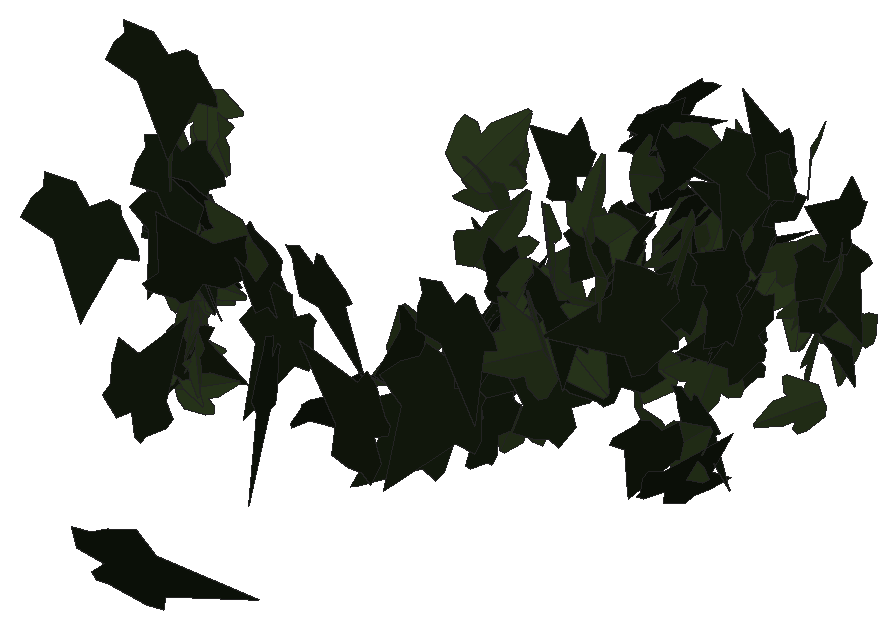
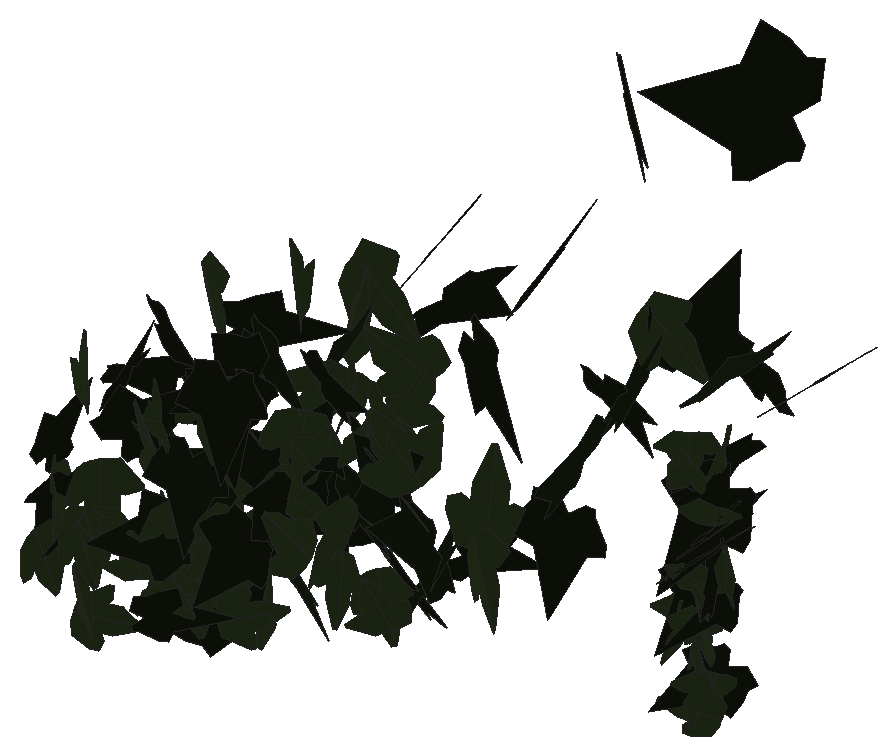
# SketchUp Ruby script. Lengths in inches.
U = 1.inch
M = Sketchup.active_model
def pt(a) = Geom::Point3d.new(a.map { |v| v * U })
def face(e, loops, mat)
  f = e.add_face(loops[0].map { |a| pt(a) })
  loops[1..].each { |l| e.add_face(l.map { |a| pt(a) }).erase! }
  f.material = f.back_material = mat if mat
  f
end
# faces: each face lists its corners as indices into pts; further lists are holes
def faces(e, pts, list, mat = nil) = list.each { |f| face(e, (f[0].is_a?(Array) ? f : [f]).map { |l| l.map { |i| pts[i] } }, mat) }
# xy, xz, yz: faces in a plane at the given z, y or x. An outline is a flat list of corners, or four numbers for a rectangle; further outlines are holes
def ring(l) = l.size == 4 ? [[l[0], l[1]], [l[2], l[1]], [l[2], l[3]], [l[0], l[3]]] : l.each_slice(2).to_a
def flat(e, list, mat, &to3) = list.each { |f| face(e, (f[0].is_a?(Array) ? f : [f]).map { |l| ring(l).map { |u, v| to3.(u, v) } }, mat) }
def xy(e, z, list, mat = nil) = flat(e, list, mat) { |x, y| [x, y, z] }
def xz(e, y, list, mat = nil) = flat(e, list, mat) { |x, z| [x, y, z] }
def yz(e, x, list, mat = nil) = flat(e, list, mat) { |y, z| [x, y, z] }
def lines(e, pts, list) = list.each { |a, b| e.add_line(pt(pts[a]), pt(pts[b])) }
# prism: a flat outline (further loops are holes) pulled along v
def prism(e, loops, v, mat = nil)
  f = face(e, loops, mat); d = Geom::Vector3d.new(v.map { |x| x * U })
  f.pushpull(f.normal.samedirection?(d) ? d.length : -d.length)
end
def box(e, o, s, mat = nil) = prism(e, [[o, [o[0] + s[0], o[1], o[2]], [o[0] + s[0], o[1] + s[1], o[2]], [o[0], o[1] + s[1], o[2]]]], [0, 0, s[2]], mat)
def at(x, y, z, deg = 0) = Geom::Transformation.translation(pt([x, y, z])) * Geom::Transformation.rotation(ORIGIN, Z_AXIS, deg.degrees)
def axes(o, x, y, z) = Geom::Transformation.new([*x, 0, *y, 0, *z, 0, *pt(o).to_a, 1])
def part(name) = M.definitions.add(name)
# library, detail: a bought-in or finely detailed component or shape, given as its bounding box
def library(name, o, s) = part(name).tap { |d| box(d.entities, o, s) }
def detail(e, o, s) = box(e.add_group.entities, o, s)
def put(e, d, t, mat = nil) = e.add_instance(d, t).tap { |i| i.material = mat if mat }
def group(e, t, mat = nil) = e.add_group.tap { |g| g.transformation = t; g.material = mat if mat }.entities
root = M.entities
M.materials.add("efeu1").color = [18, 25, 13]
M.materials.add("efeu2").color = [43, 57, 29]
c1 = part("ivyleaf_9")
p = [[1.54,2.16,1.25],[1.36,2.04,1.19],[-0.21,0.99,0.68],[-0.71,1.11,0.82],[-0.85,0.86,0.67],[-0.8,0.17,0.21],
  [-0.9,-0.01,0.1],[-0.67,-0.16,-0.02],[-0.08,-0.08,-0.05],[-0.03,-0.6,-0.4],[0.65,-0.88,-0.66],[0.83,-0.6,-0.49],
  [1.29,-0.42,-0.43],[1.8125,-0.07,-0.26],[1.21,0.44,0.15]]
faces(c1.entities,p,[[0,1,2,3,4,5,6,7,8,9,10,11,12,13,14]],"efeu1")
c2 = part("ivyleaf_10")
p = [[0,0.5,-0.03],[-0.0625,2.02,-0.43],[-0.19,2.01,-0.46],[-0.54,1.05,-0.29],[-0.52,0.625,-0.18],[-0.83,0.76,-0.28],
  [-1.16,0.64,-0.33],[-1.15,0.33,-0.24],[-0.77,-0.39,0.02],[-0.3,-0.51,0.16],[0.04,-0.48,0.23],[-0.02,2.01,-0.4375],
  [-0.06,2.01,-0.43],[0.04,-0.49,0.23],[0.67,-0.49,0.14],[1.38,0.36,-0.2],[1.375,0.51,-0.24],[0.81,0.65,-0.19],
  [0.62,0.59,-0.15],[0.6,1.09,-0.28],[0.5,1.23,-0.31]]
faces(c2.entities,p,[[0,1,2,3,4,5,6,7,8,9,10],[11,12,0,13,14,15,16,17,18,19,20]],"efeu2")
put(root,c1,axes([597.06,111.03,169.78],[0.8884,-0.27376,1.03511],[1.04614,-0.06449,-0.91492],[0.22801,1.36255,0.16467]))
put(root,c1,axes([597.32,117.23,172.98],[-0.66463,0.21669,-1.02259],[0.98764,-0.26673,-0.69844],[-0.34238,-1.19008,-0.02966]))
put(root,c1,axes([590.51,120.16,168.07],[-0.54205,0.57536,0.71293],[0.49254,-0.51545,0.79047],[0.77247,0.73239,-0.00375]))
put(root,c1,axes([597.17,121.51,169.04],[0.02116,-1.10176,0.25788],[0.00386,0.25799,1.10193],[-1.13153,-0.01973,0.00858]))
put(root,c1,axes([586.375,123.42,170.97],[-0.15788,-1.13606,0.27735],[0.27693,-0.30823,-1.10489],[1.13616,-0.08274,0.30785]))
put(root,c1,axes([590.33,123.15,170.4375],[0.56967,0.20223,0.80165],[-0.7533,-0.27424,0.60449],[0.34072,-0.94444,-0.00387]))
put(root,c1,axes([598,123.75,169.59],[-0.48576,-0.91416,0.37838],[-0.19107,-0.32691,-1.0351],[0.97074,-0.52179,-0.0144]))
put(root,c1,axes([597.72,124.3,171.68],[0.29974,-1.04193,0.1721],[0.06502,-0.16035,-1.08404],[1.05405,0.30619,0.01793]))
put(root,c2,axes([591.05,123.89,171.4375],[-0.49829,-0.14247,0.83957],[-0.81301,-0.20983,-0.51813],[0.25337,-0.95349,-0.01142]))
put(root,c1,axes([592.26,124.37,169.37],[-0.90433,-0.11689,-0.34199],[0.33902,0.04499,-0.91186],[0.12525,-0.96579,-0.00109]))
put(root,c1,axes([590.61,124.88,170.59],[0.86227,-0.73938,-0.36016],[-0.2705,0.23783,-1.13586],[0.77668,0.9037,0.00426]))
put(root,c1,axes([596.14,124.86,169.32],[0.048,0.03236,-1.17542],[-1.17289,-0.08233,-0.05016],[-0.08361,1.17352,0.02889]))
put(root,c2,axes([599.42,125.35,170.56],[-0.55467,-0.00306,0.99705],[-0.98974,-0.13623,-0.55103],[0.12053,-1.13279,0.06358]))
put(root,c1,axes([592.125,126.17,166.32],[0.24002,0.89785,0.01121],[0.00274,0.01087,-0.92938],[-0.89792,0.24003,0.00015]))
put(root,c2,axes([598.72,126.74,169.57],[-0.75092,0.65629,-0.00469],[-0.01407,-0.00897,0.99717],[0.65616,0.75088,0.01601]))
put(root,c1,axes([585.61,127.62,173.34],[-0.08041,-1.08649,0.38625],[0.35343,-0.39177,-1.02845],[1.0976,0.04655,0.35946]))
put(root,c1,axes([586,127.66,168.86],[-0.16927,-0.80439,0.33478],[-0.0648,-0.32847,-0.82199],[0.86886,-0.1812,0.00392]))
put(root,c1,axes([590.65,127.42,168.98],[0.62776,-0.88077,0.14988],[0.08887,-0.12071,-1.08159],[0.889,0.63401,0.00229]))
put(root,c1,axes([586.16,127.53,170.7],[-0.05627,-0.91989,-0.14359],[0.01497,0.14294,-0.92159],[0.93091,-0.0579,0.00614]))
put(root,c1,axes([594.01,127.92,165.32],[-0.58795,-0.5238,0.40602],[-0.29696,-0.27702,-0.78739],[0.59248,-0.65864,0.00827]))
put(root,c2,axes([585.92,127.54,171.16],[-0.11188,0.55564,-0.36798],[0.07283,-0.3607,-0.56679],[-0.66245,-0.13349,-0.00017]))
put(root,c2,axes([585.64,127.68,167.13],[-0.03748,0.01917,0.83105],[0.8178,-0.14827,0.0403],[0.14901,0.81857,-0.01216]))
put(root,c1,axes([586,127.89,168.68],[-0.0318,-0.76474,0.0772],[0.13628,-0.08165,-0.7527],[0.75645,-0.01744,0.13885]))
put(root,c1,axes([585.97,127.37,169.74],[1.0602,0.21388,-0.20249],[-0.20035,-0.0308,-1.08152],[-0.21589,1.07892,0.00927]))
put(root,c1,axes([585.77,128.15,167.96],[0.27922,-0.00862,-0.99705],[0.9911,-0.11084,0.27851],[-0.10905,-1.02946,-0.02164]))
put(root,c2,axes([585.88,127.82,169.28],[0.73001,0.22406,0.15656],[0.15003,0.04477,-0.76362],[-0.22848,0.74527,-0.00119]))
put(root,c2,axes([586.1,128.32,165.51],[0.07731,-0.15285,0.65119],[0.38199,-0.52803,-0.16929],[0.54908,0.38886,0.02608]))
put(root,c1,axes([597.76,128.48,170.02],[0.1948,-0.82397,0.50147],[0.12717,-0.48519,-0.84662],[0.95615,0.2324,0.01043]))
put(root,c2,axes([586.05,128.09,164.83],[0.42932,-0.16952,0.46116],[0.4297,-0.16744,-0.46157],[0.23827,0.60741,0.00147]))
put(root,c1,axes([585.67,128.45,168.55],[0.11192,-1.003,-0.00907],[0.23684,0.0353,-0.98045],[0.97468,0.1066,0.23928]))
put(root,c2,axes([586.08,128.42,166.22],[-0.08994,-0.52776,-0.40317],[-0.08395,-0.39455,0.53521],[-0.65881,0.12233,-0.01316]))
put(root,c2,axes([592.92,128.54,166.74],[-0.28103,-0.94674,-0.41689],[-0.06472,-0.41507,0.98622],[-1.03244,0.28373,0.05165]))
put(root,c2,axes([598.96,128.47,171.21],[-0.42654,0.23922,0.82716],[0.73699,-0.37594,0.48876],[0.44528,0.85136,-0.0166]))
put(root,c2,axes([585.95,128.09,165.59],[0.52592,-0.52848,0.06353],[-0.04314,0.04669,0.74557],[-0.53053,-0.52768,0.00235]))
put(root,c2,axes([586.09,128.04,166.2],[0.04704,-0.60915,-0.19043],[0.20875,0.19513,-0.57262],[0.60312,-0.02003,0.21305]))
put(root,c1,axes([585.7,127.71,164.83],[0.03003,-0.0198,-0.77798],[0.1901,0.75516,-0.01188],[0.75466,-0.18944,0.03395]))
put(root,c2,axes([585.88,127.95,167.17],[-0.20533,-0.35596,0.56929],[0.2824,0.49431,0.41093],[-0.60913,0.34916,-0.00139]))
put(root,c2,axes([585.81,128.08,164.51],[0.41343,0.53751,0.2657],[0.14709,0.22196,-0.6779],[-0.58128,0.43847,0.01744]))
put(root,c2,axes([585.9375,128.08,163.51],[-0.16226,-0.14107,0.62755],[0.47385,0.41144,0.21501],[-0.43495,0.50086,0.00013]))
put(root,c1,axes([585.88,127.89,167.29],[0.55625,0.56685,0.20568],[0.1443,0.14657,-0.79419],[-0.5855,0.57467,-0.00033]))
put(root,c2,axes([586.02,128.42,166.59],[0.01412,-0.02949,0.66901],[0.62415,0.24306,-0.00246],[-0.24266,0.62346,0.0326]))
put(root,c1,axes([600.49,129.09,170.24],[-0.6355,-0.23943,0.76644],[-0.72071,-0.26087,-0.67908],[0.35403,-0.96085,-0.00662]))
put(root,c2,axes([586.11,128.61,171.77],[0.50879,0.42653,0.03349],[0.02576,0.0214,-0.66393],[-0.42706,0.50945,-0.00015]))
put(root,c2,axes([586.13,128.67,171.02],[0.476,0.04723,0.42453],[0.42342,0.0317,-0.47828],[-0.05637,0.63703,-0.00768]))
put(root,c2,axes([597.88,128.32,169.19],[0.41865,0.75372,0.61853],[0.2831,0.55018,-0.86203],[-0.93302,0.50513,0.01598]))
put(root,c2,axes([586.09,128.63,166.47],[-0.03706,0.4318,0.46613],[-0.0348,0.46484,-0.43337],[-0.63444,-0.05072,-0.00346]))
put(root,c2,axes([592.17,129.65,166.68],[0.28831,-0.97294,-0.02223],[-0.00197,0.0226,-1.01475],[0.9732,0.28829,0.00453]))
put(root,c1,axes([595.1,129.25,164.93],[-0.37042,0.47129,0.68245],[-0.44921,0.51429,-0.59899],[-0.69719,-0.58177,0.02335]))
put(root,c2,axes([595.57,130.07,169.34],[0.28907,0.58516,-0.4659],[-0.20587,-0.41795,-0.65266],[-0.71909,0.35489,-0.00043]))
put(root,c1,axes([596.76,130.09,165.97],[-0.51209,-0.65297,-0.2267],[-0.10583,-0.20474,0.82878],[-0.68305,0.52126,0.04154]))
put(root,c1,axes([593.24,130.66,165.7],[0.63632,-0.642,-0.57517],[0.40104,-0.41233,0.9039],[-0.76299,-0.75214,-0.00458]))
put(root,c1,axes([598.3,130.3,167.08],[0.44154,0.0848,0.82839],[-0.82381,-0.09231,0.44855],[0.12148,-0.93417,0.03088]))
put(root,c1,axes([595.18,130.16,168.67],[-0.70253,0.34345,-0.04737],[0.04228,-0.02137,-0.78199],[-0.34411,-0.7038,0.00063]))
put(root,c1,axes([595.61,130.3,167.07],[-0.80342,0.08747,0.07003],[-0.06992,0.00484,-0.80817],[-0.08756,-0.80645,0.00275]))
put(root,c1,axes([596,130.31,167.76],[-0.59735,0.43355,-0.37409],[0.30373,-0.21839,-0.7381],[-0.48545,-0.67013,-0.00148]))
put(root,c2,axes([600.53,130.27,172.125],[0.49064,-0.8846,-0.06879],[-0.02142,0.06677,-1.01146],[0.88701,0.49092,0.01363]))
put(root,c2,axes([595.08,130.22,165.07],[-0.68788,-0.10672,0.37025],[-0.36371,-0.07037,-0.696],[0.12726,-0.77801,0.01216]))
put(root,c1,axes([594.67,130.16,167.65],[0.18212,0.79996,0.34057],[-0.08013,-0.33103,0.82042],[0.86574,-0.19892,0.00429]))
put(root,c2,axes([593.93,130.48,170.86],[-0.62573,-0.06809,-0.30328],[-0.29725,-0.06819,0.62861],[-0.09086,0.692,0.0321]))
put(root,c2,axes([597.55,130.28,168.87],[-0.85038,-0.27096,-0.00636],[0.00707,-0.00124,-0.8925],[0.27094,-0.8504,0.00333]))
put(root,c1,axes([594.78,130.17,168.62],[0.01111,-0.02404,0.76181],[-0.46805,0.6011,0.0258],[-0.60155,-0.46815,-0.006]))
put(root,c1,axes([598.77,130.55,171.12],[-0.66548,0.50808,-0.34511],[0.24692,-0.2446,-0.83625],[-0.56238,-0.70862,0.04122]))
put(root,c1,axes([596.9,130.31,167.91],[-0.21796,0.79775,-0.25818],[0.06053,-0.2511,-0.82695],[-0.8363,-0.22609,0.00743]))
put(root,c2,axes([595.65,130.66,170.8],[-0.30513,0.63443,-0.4362],[0.18684,-0.39416,-0.70399],[-0.7469,-0.35778,0.0021]))
put(root,c2,axes([593.65,130.26,171.91],[0.55823,0.35764,-0.70091],[0.59881,0.36446,0.66287],[0.5105,-0.81857,-0.0111]))
put(root,c1,axes([593.53,130,166.65],[-0.49766,0.87211,-0.31711],[-0.15723,0.27538,1.00411],[0.91456,0.5219,0.00007]))
put(root,c2,axes([593.71,130.63,169.14],[-0.33211,-0.84542,0.42958],[0.15402,0.40103,0.9083],[-0.93571,0.36607,-0.00296]))
put(root,c1,axes([599.75,131.34,169.9375],[-0.85072,0.12254,-0.19994],[0.19479,-0.0497,-0.85924],[-0.13058,-0.87248,0.02086]))
put(root,c1,axes([601.62,130.87,170.63],[-0.47725,0.01014,-0.96324],[-0.96329,-0.00248,0.47725],[0.00228,1.07498,0.01019]))
put(root,c1,axes([598.91,131.27,165.38],[0.19473,0.6141,-0.59155],[-0.16758,-0.56738,-0.64418],[-0.83604,0.25676,-0.00866]))
put(root,c2,axes([595.34,131.49,166.07],[-0.77018,0.15489,0.15891],[-0.15898,0.01531,-0.78544],[-0.15482,-0.78626,0.01601]))
put(root,c2,axes([598.79,131.79,164.6],[-0.68694,-0.1987,0.67991],[0.68297,0.06545,0.70916],[-0.1879,0.9643,0.09196]))
put(root,c1,axes([598.82,131.66,163.53],[0.56722,0.75796,0.02512],[-0.0184,-0.0176,0.94669],[0.75816,-0.5675,0.00419]))
put(root,c2,axes([593.79,131.9,171.3125],[0.13378,-0.03188,0.70052],[-0.69146,0.1127,0.13718],[-0.11672,-0.70422,-0.00976]))
put(root,c1,axes([595.57,131.88,171.5625],[-0.25118,0.27057,0.71602],[-0.48676,0.52511,-0.36919],[-0.59072,-0.54775,-0.00024]))
put(root,c2,axes([593.36,132,165.41],[0.55969,0.33852,-0.29635],[0.2512,0.15728,0.65409],[0.37324,-0.61347,0.00416]))
put(root,c1,axes([596.17,132.3125,165.99],[-0.4261,0.54584,0.35352],[-0.20169,0.29088,-0.69223],[-0.61825,-0.47108,-0.01782]))
put(root,c1,axes([600.9,132.62,168.37],[-0.76474,0.40091,0.35041],[-0.33357,0.11726,-0.86216],[-0.41502,-0.83299,0.04728]))
put(root,c2,axes([594.72,132.06,167.91],[-0.13792,0.60092,0.72541],[-0.22409,0.69116,-0.61515],[-0.91493,-0.25987,0.04132]))
put(root,c1,axes([598.53,133.06,165.28],[0.48761,-0.66804,0.15474],[0.07487,-0.13687,-0.82683],[0.68163,0.49292,-0.01988]))
put(root,c1,axes([600.26,132.69,168.71],[-0.6034,0.72742,-0.05195],[0.04413,-0.03089,-0.945],[-0.72794,-0.60484,-0.01422]))
put(root,c2,axes([595.81,133.43,169.12],[0.46055,0.2555,-0.64393],[-0.58406,-0.27265,-0.52591],[-0.37258,0.74325,0.02844]))
put(root,c2,axes([595.48,132.96,167.17],[0.15121,-0.72012,0.44867],[-0.0207,0.45248,0.73319],[-0.8482,-0.13942,0.06209]))
put(root,c2,axes([595.24,132.75,169.71],[0.02597,0.62244,-0.59236],[0.02925,0.59165,0.62297],[0.85876,-0.03898,-0.0033]))
put(root,c2,axes([596.36,133.42,164.6875],[-0.56721,0.43189,0.2144],[0.15782,-0.14651,0.71264],[0.45562,0.58842,0.02007]))
put(root,c1,axes([595.43,133.33,169.27],[0.03439,-0.62455,-0.66184],[-0.04193,0.66052,-0.62549],[0.90903,0.05409,-0.00381]))
put(root,c2,axes([596.64,134.45,167.57],[-0.01213,0.05432,0.9255],[0.19695,-0.9043,0.05565],[0.90593,0.19732,0.0003]))
put(root,c2,axes([596.64,133.2,171.33],[-0.18382,0.33024,0.71417],[-0.33552,0.63048,-0.3779],[-0.7117,-0.38253,-0.0063]))
put(root,c2,axes([596.75,134.08,165.22],[-0.12166,-0.06904,-0.71395],[-0.67633,-0.23015,0.13751],[-0.23891,0.6867,-0.0257]))
put(root,c2,axes([598.42,133.96,165.8],[-0.61158,-0.49514,0.26653],[-0.18979,-0.18893,-0.78646],[0.52932,-0.63982,0.02596]))
put(root,c2,axes([597.91,133.89,167.57],[-0.13835,-0.78084,-0.30632],[0.19811,0.27125,-0.78094],[0.81505,-0.19848,0.13783]))
put(root,c1,axes([597.22,134.61,168.54],[0.37157,-0.36728,-0.67008],[0.73435,-0.03437,0.42604],[-0.21126,-0.76543,0.3024]))
put(root,c1,axes([596.37,133.64,172.27],[0.47089,0.40324,0.61769],[0.43033,0.44504,-0.61858],[-0.59914,0.63657,0.04118]))
put(root,c1,axes([599.27,134.78,172],[-0.57169,-0.68993,-0.10118],[0.14804,0.00777,-0.88944],[0.68142,-0.58053,0.10834]))
put(root,c2,axes([597.17,134.42,169.01],[-0.18623,-0.83777,0.00724],[-0.00128,-0.00714,-0.85822],[0.8378,-0.18623,0.0003]))
put(root,c1,axes([596.96,134.23,172],[0.53231,0.36812,-0.645],[-0.53477,-0.36065,-0.64718],[-0.51532,0.75452,0.00534]))
put(root,c1,axes([597.14,133.97,169.11],[-0.08396,0.74638,-0.18721],[-0.02122,0.186,0.75109],[0.76921,0.0866,0.00029]))
put(root,c1,axes([599.39,134.7,170.09],[-0.83289,0.18831,-0.16249],[0.15602,-0.04672,-0.85384],[-0.19371,-0.84731,0.01097]))
put(root,c2,axes([598.12,135.09,167.51],[-0.18411,0.35572,-0.90335],[0.44165,-0.78812,-0.40036],[-0.8646,-0.47834,-0.01215]))
put(root,c2,axes([596.86,134.625,171.99],[-0.7109,-0.56861,0.02747],[-0.02122,-0.01744,-0.91032],[0.56887,-0.71121,0.00037]))
put(root,c1,axes([599.39,135.14,170.11],[0.02286,0.00023,0.88107],[-0.83956,-0.26734,0.02185],[0.26725,-0.83984,-0.00672]))
put(root,c2,axes([598.76,134.85,169.63],[0.55386,-0.69026,0.08885],[-0.02347,0.09496,0.88405],[-0.69556,-0.55284,0.04092]))
put(root,c2,axes([597.24,135.25,167.98],[-0.42311,-0.28697,0.47653],[-0.38205,-0.28524,-0.511],[0.40431,-0.56985,0.01581]))
put(root,c2,axes([597.89,135.42,166.21],[0.46746,0.42898,-0.34585],[-0.26401,-0.22373,-0.63435],[-0.48367,0.53672,0.012]))
put(root,c1,axes([599.55,135.36,171.51],[-0.08898,-0.76389,0.342],[0.08208,0.3343,0.76805],[-0.83291,0.11455,0.03916]))
put(root,c2,axes([600.21,135.7,164.77],[-0.1122,-0.17915,0.69474],[-0.33045,-0.61125,-0.21099],[0.63683,-0.34874,0.01292]))
put(root,c1,axes([596.3125,134.84,172.57],[0.10945,0.89281,-0.02684],[-0.00342,-0.02662,-0.89949],[-0.8932,0.1095,0.00016]))
put(root,c2,axes([598.24,135.25,166.19],[-0.15495,-0.02959,0.67515],[-0.67466,-0.03346,-0.1563],[0.03926,-0.69189,-0.02131]))
put(root,c1,axes([598.16,135.78,165.5],[-0.48909,-0.15683,0.60953],[-0.57734,-0.19559,-0.51358],[0.25061,-0.75663,0.00642]))
put(root,c2,axes([597.71,135.86,171.4375],[0.2711,-0.16793,0.71501],[0.67296,-0.24852,-0.31352],[0.29422,0.72317,0.05829]))
put(root,c1,axes([597.19,135.18,170.16],[0.07093,0.88055,0.03894],[0.01962,0.03748,-0.88325],[-0.8812,0.07172,-0.01653]))
put(root,c2,axes([597.27,135.8,169.03],[0.35928,0.69517,-0.33859],[-0.21189,-0.27055,-0.78031],[-0.74364,0.41294,0.05875]))
put(root,c2,axes([599.98,136.18,171.67],[0.17159,-0.46643,-0.6223],[0.21069,-0.58556,0.49698],[-0.74862,-0.27171,-0.00277]))
put(root,c2,axes([596.06,135.33,168.73],[-0.16289,-0.55678,-0.65136],[0.23507,0.60855,-0.57897],[0.82402,-0.28367,0.03641]))
put(root,c2,axes([599.75,135.79,169.08],[-0.42738,-0.72903,-0.05451],[0.01659,0.05346,-0.84497],[0.73088,-0.42752,-0.0127]))
put(root,c2,axes([599.8,135.95,167.91],[0.73259,0.3693,-0.03012],[-0.02563,-0.01606,-0.8204],[-0.36964,0.73303,-0.0028]))
put(root,c2,axes([600.08,136.2,167.61],[-0.15527,-0.79477,0.13566],[-0.05441,-0.12751,-0.80929],[0.80442,-0.16203,-0.02856]))
put(root,c1,axes([600.82,136.54,169.75],[-0.00331,0.10101,0.758],[-0.38963,-0.65246,0.08525],[0.65799,-0.38584,0.05429]))
put(root,c1,axes([600.27,136.22,167.66],[0.31837,-0.74494,-0.13559],[-0.01672,0.14013,-0.80918],[0.757,0.31639,0.03915]))
put(root,c1,axes([600.48,136.19,168.95],[0.08507,-0.69083,-0.44087],[-0.03483,0.43979,-0.69586],[0.81878,0.09048,0.0162]))
put(root,c2,axes([601.09,136.55,166.96],[-0.15358,-0.74557,0.25804],[0.05726,-0.27272,-0.75392],[0.78688,-0.12567,0.10523]))
put(root,c1,axes([597.36,135.76,168.06],[0.53722,0.08088,0.62448],[0.46102,0.50863,-0.46248],[-0.42893,0.64798,0.28507]))
put(root,c2,axes([599.85,136.48,166.29],[0.37418,-0.72575,0.07772],[0.06148,-0.05569,-0.81601],[0.7273,0.37809,0.02899]))
put(root,c2,axes([600.86,136.05,168.9],[0.15651,-0.64294,-0.52047],[-0.10722,0.50947,-0.66159],[0.82022,0.18928,0.01283]))
put(root,c1,axes([594.83,135.86,168.92],[0.37633,0.62563,0.35037],[0.1791,0.30113,-0.73009],[-0.69432,0.41677,0.00157]))
put(root,c2,axes([598,136.33,167.17],[0.56855,0.31019,-0.12846],[0.11169,0.0635,0.64766],[0.31661,-0.57941,0.00221]))
